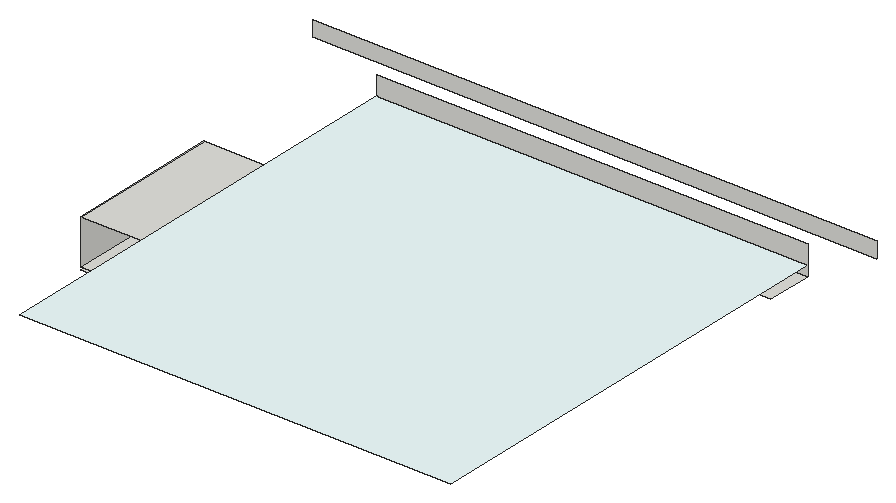
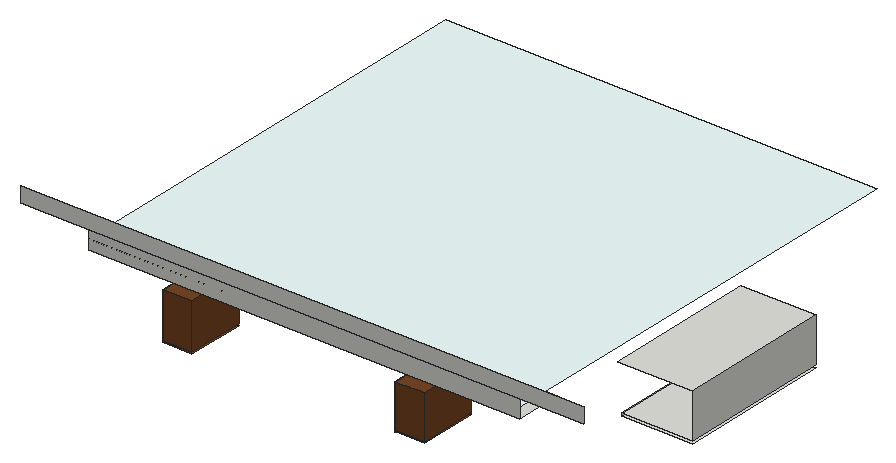
# SketchUp Ruby script. Lengths in inches.
U = 1.inch
M = Sketchup.active_model
def pt(a) = Geom::Point3d.new(a.map { |v| v * U })
def face(e, loops, mat)
  f = e.add_face(loops[0].map { |a| pt(a) })
  loops[1..].each { |l| e.add_face(l.map { |a| pt(a) }).erase! }
  f.material = f.back_material = mat if mat
  f
end
# faces: each face lists its corners as indices into pts; further lists are holes
def faces(e, pts, list, mat = nil) = list.each { |f| face(e, (f[0].is_a?(Array) ? f : [f]).map { |l| l.map { |i| pts[i] } }, mat) }
# xy, xz, yz: faces in a plane at the given z, y or x. An outline is a flat list of corners, or four numbers for a rectangle; further outlines are holes
def ring(l) = l.size == 4 ? [[l[0], l[1]], [l[2], l[1]], [l[2], l[3]], [l[0], l[3]]] : l.each_slice(2).to_a
def flat(e, list, mat, &to3) = list.each { |f| face(e, (f[0].is_a?(Array) ? f : [f]).map { |l| ring(l).map { |u, v| to3.(u, v) } }, mat) }
def xy(e, z, list, mat = nil) = flat(e, list, mat) { |x, y| [x, y, z] }
def xz(e, y, list, mat = nil) = flat(e, list, mat) { |x, z| [x, y, z] }
def yz(e, x, list, mat = nil) = flat(e, list, mat) { |y, z| [x, y, z] }
def lines(e, pts, list) = list.each { |a, b| e.add_line(pt(pts[a]), pt(pts[b])) }
# prism: a flat outline (further loops are holes) pulled along v
def prism(e, loops, v, mat = nil)
  f = face(e, loops, mat); d = Geom::Vector3d.new(v.map { |x| x * U })
  f.pushpull(f.normal.samedirection?(d) ? d.length : -d.length)
end
def box(e, o, s, mat = nil) = prism(e, [[o, [o[0] + s[0], o[1], o[2]], [o[0] + s[0], o[1] + s[1], o[2]], [o[0], o[1] + s[1], o[2]]]], [0, 0, s[2]], mat)
def at(x, y, z, deg = 0) = Geom::Transformation.translation(pt([x, y, z])) * Geom::Transformation.rotation(ORIGIN, Z_AXIS, deg.degrees)
def axes(o, x, y, z) = Geom::Transformation.new([*x, 0, *y, 0, *z, 0, *pt(o).to_a, 1])
def part(name) = M.definitions.add(name)
# library, detail: a bought-in or finely detailed component or shape, given as its bounding box
def library(name, o, s) = part(name).tap { |d| box(d.entities, o, s) }
def detail(e, o, s) = box(e.add_group.entities, o, s)
def put(e, d, t, mat = nil) = e.add_instance(d, t).tap { |i| i.material = mat if mat }
def group(e, t, mat = nil) = e.add_group.tap { |g| g.transformation = t; g.material = mat if mat }.entities
root = M.entities
M.materials.add("[0092_Azure]").color = [240, 255, 255]
M.materials.add("[Color M08]").color = [30, 30, 30]
M.materials.add("[Wood Veneer 01]").color = [120, 70, 37]
c1 = library("10 (1)",[26.65,-5.45,122.92],[1.37,1.38,0.36])
c2 = library("Group\#131",[-0.5,-0.5,0],[91.72,99.22,1.125])
c3 = library("Group\#127",[-0.5,-0.5,0],[1.6875,13.62,0.5625])
c4 = library("Group\#130",[-0.5,-0.5,0],[1.6875,13.62,0.5625])
c5 = library("Spot Light",[-5.1,-5.1,-11.05],[10.2,10.2,11.05])
c6 = library("Group\#122",[0,0,0],[7,7.02,10])
c7 = library("Group\#119",[0,0,0],[7,7.02,10])
c8 = library("Stocked cup rack",[0,0,0],[12.28,12.62,7.74])
xy(root,89.07,[[0.8125,335.99,28.4375,396.27]])
xy(root,89.71,[[154.0625,426.125,165.5625,448.75]],"[Wood Veneer 01]")
xy(root,90.07,[[0.8125,335.99,28.4375,396.27]])
xy(root,90.4,[[154.0625,426.125,165.5625,448.75]])
xy(root,90.4,[[63.375,426.125,74.1875,448.75],[74.1875,426.125,74.78,448.75]],"[Wood Veneer 01]")
xy(root,90.96,[[63.375,426.125,74.1875,448.75],[74.1875,426.125,74.78,448.75]])
xy(root,107.6,[[0.8125,335.99,30,396.27]])
xy(root,107.92,[[63.375,426.125,74.78,448.75]],"[Wood Veneer 01]")
xy(root,108.12,[[154.0625,426.125,165.5625,448.75]],"[Wood Veneer 01]")
xy(root,108.59,[[75.375,422.75,94.92,422.75,94.92,423.05,95.22,423.05,95.22,422.75,114.47,422.75,114.47,423.05,114.77,423.05,114.77,422.75,134.02,422.75,134.02,423.05,134.32,423.05,134.32,422.75,153.5625,422.75,153.5625,426.125,155.1875,426.125,155.1875,444.125,74.1875,444.125,74.1875,426.125,75.375,426.125],[30,426.125,74.1875,444.125],[155.1875,426.125,198,444.125]])
xy(root,108.59,[[77.14,369.75,77.83,382.37],[150.17,369.75,150.86,382.37]],"[0092_Azure]")
xy(root,108.59,[[77.14,357.125,77.83,369.75],[150.17,357.125,150.86,369.75],[77.08,382.37,77.83,390.24],[150.17,382.37,150.86,390.87]],"[Color M08]")
xy(root,109.47,[[67.14,308.76,68.64,406.99],[159.36,308.76,160.86,406.99]],"[0092_Azure]")
xy(root,109.59,[[56.1,354.125,55.32,354.2,54.59,354.48,53.95,354.94,53.45,355.54,53.13,356.25,53,357.03,53.08,357.81,53.35,358.54,53.81,359.18,54.42,359.67,55.13,360,55.9,360.125,56.68,360.05,57.41,359.77,58.05,359.31,58.55,358.71,58.87,358,59,357.22,58.92,356.44,58.65,355.71,58.19,355.07,57.58,354.58,56.87,354.25],[172,354.125,171.22,354.23,170.5,354.53,169.88,355,169.4,355.625,169.1,356.35,169,357.125,169.1,357.9,169.4,358.625,169.88,359.25,170.5,359.72,171.22,360.02,172,360.125,172.78,360.02,173.5,359.72,174.12,359.25,174.6,358.625,174.9,357.9,175,357.125,174.9,356.35,174.6,355.625,174.12,355,173.5,354.53,172.78,354.23],[114,415.125,113.22,415.23,112.5,415.53,111.88,416,111.4,416.625,111.1,417.35,111,418.125,111.1,418.9,111.4,419.625,111.88,420.25,112.5,420.72,113.22,421.02,114,421.125,114.78,421.02,115.5,420.72,116.12,420.25,116.6,419.625,116.9,418.9,117,418.125,116.9,417.35,116.6,416.625,116.12,416,115.5,415.53,114.78,415.23],[172,415.125,171.22,415.23,170.5,415.53,169.88,416,169.4,416.625,169.1,417.35,169,418.125,169.1,418.9,169.4,419.625,169.88,420.25,170.5,420.72,171.22,421.02,172,421.125,172.78,421.02,173.5,420.72,174.12,420.25,174.6,419.625,174.9,418.9,175,418.125,174.9,417.35,174.6,416.625,174.12,416,173.5,415.53,172.78,415.23],[56.24,415.45,55.53,415.48,54.87,415.6875,54.27,416.07,53.8,416.58,53.47,417.2,53.32,417.89,53.35,418.59,53.5625,419.26,53.94,419.85,54.46,420.33,55.08,420.65,55.76,420.8,56.47,420.77,57.13,420.5625,57.73,420.18,58.2,419.67,58.53,419.05,58.68,418.36,58.65,417.66,58.4375,416.99,58.06,416.4,57.54,415.92,56.92,415.6]],"[0092_Azure]")
xy(root,110.59,[[[64.57,304.7,163.43,409.55],[68.64,308.76,159.36,406.99]]],"[0092_Azure]")
xy(root,112.59,[[30,270.125,198,444.125]],"[0092_Azure]")
xz(root,382.37,[[77.14,108.03,77.83,108.59],[150.17,108.03,150.86,108.59]],"[0092_Azure]")
xz(root,406.99,[[67.14,108.59,67.14,109.47,68.64,109.47,68.64,110.59,159.36,110.59,159.36,109.47,160.86,109.47,160.86,108.59]],"[0092_Azure]")
xz(root,409.55,[[64.57,108.59,163.43,110.59]],"[0092_Azure]")
xz(root,426.125,[[63.375,90.4,74.78,90.96]],"[Wood Veneer 01]")
xz(root,444.125,[[30,108.59,198,120]])
xz(root,444.125,[[30,108.59,198,112.59]],"[0092_Azure]")
xz(root,448.75,[[154.0625,90.4,165.5625,108.12],[63.375,90.96,74.78,107.92]],"[Wood Veneer 01]")
xz(root,450.125,[[0,120,220,126]])
yz(root,0.8125,[[335.99,90.07,396.27,107.6]])
yz(root,28.4375,[[335.99,89.07,396.27,90.07]])
yz(root,63.375,[[426.125,90.96,448.75,107.92]],"[Wood Veneer 01]")
yz(root,64.57,[[304.7,108.59,409.55,110.59]],"[0092_Azure]")
yz(root,74.78,[[426.125,90.96,448.75,107.92]],"[Wood Veneer 01]")
yz(root,154.0625,[[426.125,90.4,448.75,108.12]],"[Wood Veneer 01]")
yz(root,163.43,[[304.7,108.59,409.55,110.59]],"[0092_Azure]")
yz(root,165.5625,[[426.125,90.4,448.75,108.12]],"[Wood Veneer 01]")
p = [[53,357.03,108.59],[53.08,357.81,108.59],[53.08,357.81,109.59],[53,357.03,109.59],[169,357.125,108.59],[169.1,357.9,108.59],
  [169.1,357.9,109.59],[169,357.125,109.59],[174.9,357.9,108.59],[175,357.125,108.59],[175,357.125,109.59],[174.9,357.9,109.59],
  [58.87,358,108.59],[59,357.22,108.59],[59,357.22,109.59],[58.87,358,109.59],[53.35,358.54,108.59],[53.35,358.54,109.59],
  [169.4,358.625,108.59],[169.4,358.625,109.59],[174.6,358.625,108.59],[174.6,358.625,109.59],[58.55,358.71,108.59],[58.55,358.71,109.59],
  [53.81,359.18,108.59],[53.81,359.18,109.59],[169.88,359.25,108.59],[169.88,359.25,109.59],[174.12,359.25,108.59],[174.12,359.25,109.59],
  [58.05,359.31,108.59],[58.05,359.31,109.59],[54.42,359.67,108.59],[54.42,359.67,109.59],[170.5,359.72,108.59],[170.5,359.72,109.59],
  [173.5,359.72,108.59],[173.5,359.72,109.59],[57.41,359.77,108.59],[57.41,359.77,109.59],[55.13,360,108.59],[55.13,360,109.59],
  [171.22,360.02,108.59],[171.22,360.02,109.59],[172.78,360.02,108.59],[172.78,360.02,109.59],[56.68,360.05,108.59],[56.68,360.05,109.59],
  [55.9,360.125,108.59],[55.9,360.125,109.59],[172,360.125,108.59],[172,360.125,109.59],[114,415.125,108.59],[113.22,415.23,108.59],
  [113.22,415.23,109.59],[114,415.125,109.59],[114.78,415.23,108.59],[114.78,415.23,109.59],[172,415.125,108.59],[171.22,415.23,108.59],
  [171.22,415.23,109.59],[172,415.125,109.59],[172.78,415.23,108.59],[172.78,415.23,109.59],[112.5,415.53,108.59],[112.5,415.53,109.59],
  [115.5,415.53,108.59],[115.5,415.53,109.59],[170.5,415.53,108.59],[170.5,415.53,109.59],[173.5,415.53,108.59],[173.5,415.53,109.59],
  [56.24,415.45,108.59],[55.53,415.48,108.59],[55.53,415.48,109.59],[56.24,415.45,109.59],[56.92,415.6,108.59],[56.92,415.6,109.59],
  [54.87,415.6875,108.59],[54.87,415.6875,109.59],[111.88,416,108.59],[111.88,416,109.59],[116.12,416,108.59],[116.12,416,109.59],
  [169.88,416,108.59],[169.88,416,109.59],[174.12,416,108.59],[174.12,416,109.59],[57.54,415.92,108.59],[57.54,415.92,109.59],
  [54.27,416.07,108.59],[54.27,416.07,109.59],[58.06,416.4,108.59],[58.06,416.4,109.59],[111.4,416.625,108.59],[111.4,416.625,109.59],
  [116.6,416.625,108.59],[116.6,416.625,109.59],[169.4,416.625,108.59],[169.4,416.625,109.59],[174.6,416.625,108.59],[174.6,416.625,109.59],
  [53.8,416.58,108.59],[53.8,416.58,109.59],[58.4375,416.99,108.59],[58.4375,416.99,109.59],[53.47,417.2,108.59],[53.47,417.2,109.59],
  [111.1,417.35,108.59],[111.1,417.35,109.59],[116.9,417.35,108.59],[116.9,417.35,109.59],[169.1,417.35,108.59],[169.1,417.35,109.59],
  [174.9,417.35,108.59],[174.9,417.35,109.59],[58.65,417.66,108.59],[58.65,417.66,109.59],[53.32,417.89,108.59],[53.32,417.89,109.59],
  [111,418.125,108.59],[111,418.125,109.59],[117,418.125,108.59],[117,418.125,109.59],[169,418.125,108.59],[169,418.125,109.59],
  [175,418.125,108.59],[175,418.125,109.59],[58.68,418.36,108.59],[58.68,418.36,109.59],[53.35,418.59,108.59],[53.35,418.59,109.59],
  [111.1,418.9,108.59],[111.1,418.9,109.59],[116.9,418.9,108.59],[116.9,418.9,109.59],[169.1,418.9,108.59],[169.1,418.9,109.59],
  [174.9,418.9,108.59],[174.9,418.9,109.59],[58.53,419.05,108.59],[58.53,419.05,109.59],[53.5625,419.26,108.59],[53.5625,419.26,109.59],
  [111.4,419.625,108.59],[111.4,419.625,109.59],[116.6,419.625,108.59],[116.6,419.625,109.59],[169.4,419.625,108.59],[169.4,419.625,109.59],
  [174.6,419.625,108.59],[174.6,419.625,109.59],[58.2,419.67,108.59],[58.2,419.67,109.59],[53.94,419.85,108.59],[53.94,419.85,109.59],
  [111.88,420.25,108.59],[111.88,420.25,109.59],[116.12,420.25,108.59],[116.12,420.25,109.59],[169.88,420.25,108.59],[169.88,420.25,109.59],
  [174.12,420.25,108.59],[174.12,420.25,109.59],[57.73,420.18,108.59],[57.73,420.18,109.59],[54.46,420.33,108.59],[54.46,420.33,109.59],
  [57.13,420.5625,108.59],[57.13,420.5625,109.59],[112.5,420.72,108.59],[112.5,420.72,109.59],[115.5,420.72,108.59],[115.5,420.72,109.59],
  [170.5,420.72,108.59],[170.5,420.72,109.59],[173.5,420.72,108.59],[173.5,420.72,109.59],[55.08,420.65,108.59],[55.08,420.65,109.59],
  [56.47,420.77,108.59],[56.47,420.77,109.59],[55.76,420.8,108.59],[55.76,420.8,109.59],[113.22,421.02,108.59],[113.22,421.02,109.59],
  [114.78,421.02,108.59],[114.78,421.02,109.59],[171.22,421.02,108.59],[171.22,421.02,109.59],[172.78,421.02,108.59],[172.78,421.02,109.59],
  [114,421.125,108.59],[114,421.125,109.59],[172,421.125,108.59],[172,421.125,109.59]]
faces(root,p,[[0,1,2,3],[4,5,6,7],[8,9,10,11],[12,13,14,15],[1,16,17,2],[5,18,19,6],[20,8,11,21],[22,12,15,23],
  [16,24,25,17],[18,26,27,19],[28,20,21,29],[30,22,23,31],[24,32,33,25],[26,34,35,27],[36,28,29,37],[38,30,31,39],
  [32,40,41,33],[34,42,43,35],[44,36,37,45],[46,38,39,47],[40,48,49,41],[48,46,47,49],[42,50,51,43],[50,44,45,51],
  [52,53,54,55],[56,52,55,57],[58,59,60,61],[62,58,61,63],[53,64,65,54],[66,56,57,67],[59,68,69,60],[70,62,63,71],
  [72,73,74,75],[76,72,75,77],[73,78,79,74],[64,80,81,65],[82,66,67,83],[68,84,85,69],[86,70,71,87],[88,76,77,89],
  [78,90,91,79],[92,88,89,93],[80,94,95,81],[96,82,83,97],[84,98,99,85],[100,86,87,101],[90,102,103,91],[104,92,93,105],
  [102,106,107,103],[94,108,109,95],[110,96,97,111],[98,112,113,99],[114,100,101,115],[116,104,105,117],[106,118,119,107],[108,120,121,109],
  [122,110,111,123],[112,124,125,113],[126,114,115,127],[128,116,117,129],[118,130,131,119],[120,132,133,121],[134,122,123,135],[124,136,137,125],
  [138,126,127,139],[140,128,129,141],[130,142,143,131],[132,144,145,133],[146,134,135,147],[136,148,149,137],[150,138,139,151],[152,140,141,153],
  [142,154,155,143],[144,156,157,145],[158,146,147,159],[148,160,161,149],[162,150,151,163],[164,152,153,165],[154,166,167,155],[168,164,165,169],
  [156,170,171,157],[172,158,159,173],[160,174,175,161],[176,162,163,177],[166,178,179,167],[180,168,169,181],[178,182,183,179],[170,184,185,171],
  [186,172,173,187],[174,188,189,175],[190,176,177,191],[182,180,181,183],[184,192,193,185],[192,186,187,193],[188,194,195,189],[194,190,191,195]],"[0092_Azure]")
put(root,c1,axes([46.75,376.03,-868.89],[4.58872,0,0],[0,3.9672,0],[0,0,7.9518]),"[0092_Azure]")
put(root,c1,axes([-69.125,376.03,-868.89],[4.58872,0,0],[0,3.9672,0],[0,0,7.9518]),"[0092_Azure]")
put(root,c2,at(68.64,308.76,109.47),"[0092_Azure]")
put(root,c3,at(150.17,369.75,108.03),"[0092_Azure]")
put(root,c4,at(77.14,369.75,108.03),"[0092_Azure]")
put(root,c1,axes([-74.8,439.42,-1021],[4.79002,0,0],[0,4.58212,0],[0,0,9.18432]),"[0092_Azure]")
put(root,c1,axes([-16.8,440,-1021],[4.79002,0,0],[0,4.58212,0],[0,0,9.18432]),"[0092_Azure]")
put(root,c1,axes([46.41,437.17,-868.875],[4.58872,0,0],[0,3.9672,0],[0,0,7.9518]),"[0092_Azure]")
put(root,c5,axes([55.55,419.75,108.42],[0.3,0,0],[0,0.3,0],[0,0,0.3]))
put(root,c5,axes([114.02,419.9375,109.59],[0.3,0,0],[0,0.3,0],[0,0,0.3]))
put(root,c5,axes([173.02,419.9375,109.59],[0.3,0,0],[0,0.3,0],[0,0,0.3]))
put(root,c6,axes([68.78,426.125,90.96],[0.48,0,0],[0,0.48,0],[0,0,0.48]))
put(root,c7,axes([64.21,426.125,90.96],[0.5,0,0],[0,0.5,0],[0,0,0.5]))
put(root,c8,axes([155.3,426.125,90.4],[0.77,0,0],[0,0.77,0],[0,0,0.77]))
